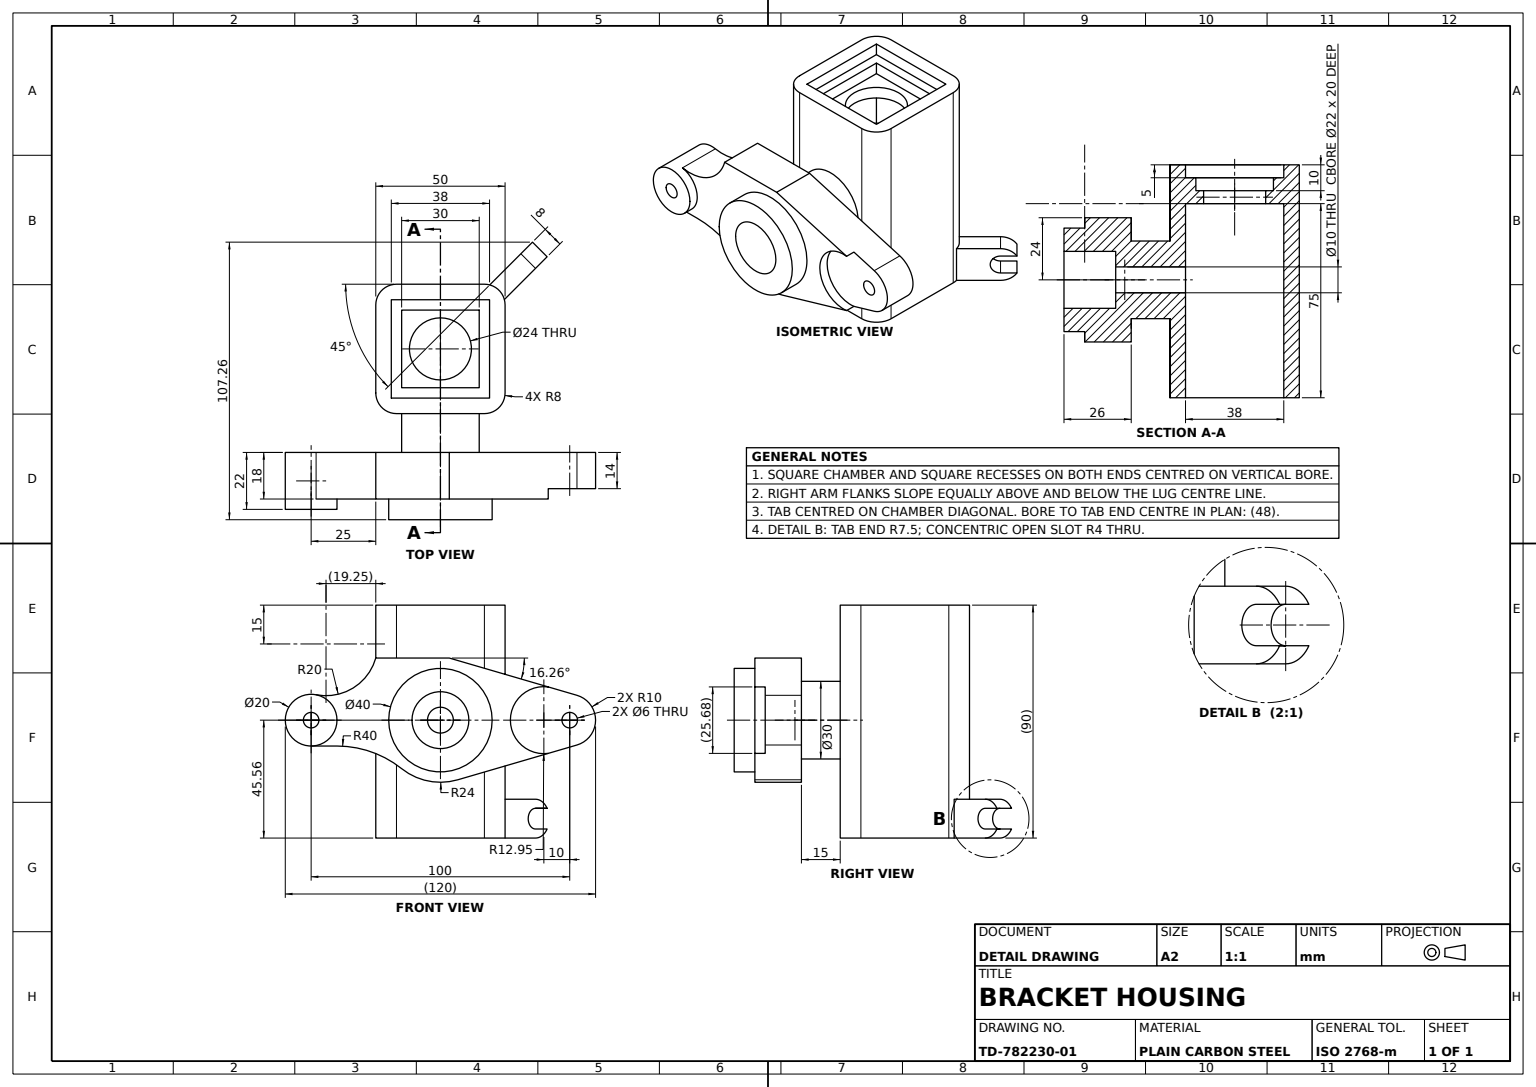
solid
v1 (25,0,17)
v2 (25,0,-17)
e1 v1 v2 LINE
v3 (25,-90,17)
e2 v3 v1 LINE
v4 (25,-90,-17)
e3 v3 v4 LINE
e4 v4 v2 LINE
face PLANE(AX(P(25,-90,17),D(1,0,0),D(0,0,-1))) [-e1 -e2 e3 e4]
v5 (-11,-44.442853,46)
v6 (-11,-44.442853,66)
e5 v5 v6 LINE
v7 (11,-44.442853,66)
e6 v6 v7 CIRCLE(AX(P(0,-44.442853,66),D(0,0,1),D(1,0,0)),11)
v8 (11,-44.442853,46)
e7 v8 v7 LINE
e8 v5 v8 CIRCLE(AX(P(0,-44.442853,46),D(0,0,1),D(1,0,0)),11)
face CYL(AX(P(0,-44.442853,66),D(0,0,1),D(1,0,0)),11) rev [e5 e6 -e7 -e8]
v9 (47,-44.442853,40)
v10 (53,-44.442853,40)
e9 v9 v10 CIRCLE(AX(P(50,-44.442853,40),D(0,0,1),D(1,0,0)),3)
v11 (47,-44.442853,54)
e10 v11 v9 LINE
v12 (53,-44.442853,54)
e11 v11 v12 CIRCLE(AX(P(50,-44.442853,54),D(0,0,1),D(1,0,0)),3)
e12 v12 v10 LINE
face CYL(AX(P(50,-44.442853,54),D(0,0,-1),D(-1,0,0)),3) rev [-e9 -e10 e11 e12]
v13 (-19,-90,-19)
v14 (19,-90,-19)
e13 v13 v14 LINE
v15 (19,-15,-19)
e14 v14 v15 LINE
v16 (-19,-15,-19)
e15 v16 v15 LINE
e16 v13 v16 LINE
face PLANE(AX(P(-19,-90,-19),D(0,0,1),D(1,0,0))) [e13 e14 -e15 -e16]
v17 (-19,0,19)
v18 (19,0,19)
e17 v17 v18 LINE
v19 (19,-5,19)
e18 v19 v18 LINE
v20 (-19,-5,19)
e19 v20 v19 LINE
e20 v20 v17 LINE
face PLANE(AX(P(-19,-5,19),D(0,0,1),D(1,0,0))) rev [e17 -e18 -e19 e20]
v21 (31.112698,-75,-36.769553)
v22 (19.070552,-75,-24.727407)
e21 v21 v22 LINE
v23 (24.727407,-75,-19.070552)
e22 v23 v22 CIRCLE(AX(P(17,-75,-17),D(0,1,0),D(1,0,0)),8)
v24 (36.769553,-75,-31.112698)
e23 v24 v23 LINE
e24 v24 v21 LINE
face PLANE(AX(P(36.769553,-75,-31.112698),D(0,-1,0),D(1,0,0))) rev [e21 -e22 -e23 e24]
v25 (41.255642,-78.5,-35.598788)
e25 v25 v24 CIRCLE(AX(P(36.769553,-82.5,-31.112698),D(0.707106781,0,0.707106781),D(0.707106781,0,-0.707106781)),7.5)
v26 (24.727407,-90,-19.070552)
e26 v23 v26 LINE
v27 (36.769553,-90,-31.112698)
e27 v26 v27 LINE
v28 (41.255642,-86.5,-35.598788)
e28 v27 v28 CIRCLE(AX(P(36.769553,-82.5,-31.112698),D(0.707106781,0,0.707106781),D(0.707106781,0,-0.707106781)),7.5)
v29 (36.769553,-86.5,-31.112698)
e29 v28 v29 LINE
v30 (33.941125,-82.5,-28.284271)
e30 v29 v30 CIRCLE(AX(P(36.769553,-82.5,-31.112698),D(-0.707106781,0,-0.707106781),D(0.707106781,0,-0.707106781)),4)
v31 (36.769553,-78.5,-31.112698)
e31 v30 v31 CIRCLE(AX(P(36.769553,-82.5,-31.112698),D(-0.707106781,0,-0.707106781),D(0.707106781,0,-0.707106781)),4)
e32 v31 v25 LINE
face PLANE(AX(P(36.769553,-82.5,-31.112698),D(0.707106781,0,0.707106781),D(0.707106781,0,-0.707106781))) [e25 e23 e26 e27 e28 e29 e30 e31 e32]
v32 (-53,-44.442853,40)
v33 (-47,-44.442853,40)
e33 v32 v33 CIRCLE(AX(P(-50,-44.442853,40),D(0,0,1),D(1,0,0)),3)
v34 (-53,-44.442853,62)
e34 v34 v32 LINE
v35 (-47,-44.442853,62)
e35 v34 v35 CIRCLE(AX(P(-50,-44.442853,62),D(0,0,1),D(1,0,0)),3)
e36 v35 v33 LINE
face CYL(AX(P(-50,-44.442853,62),D(0,0,-1),D(-1,0,0)),3) rev [-e33 -e34 e35 e36]
v36 (-15,-10,15)
v37 (-15,-10,-15)
e37 v36 v37 LINE
v38 (-15,-5,-15)
e38 v37 v38 LINE
v39 (-15,-5,15)
e39 v38 v39 LINE
e40 v36 v39 LINE
face PLANE(AX(P(-15,-10,15),D(1,0,0),D(0,0,-1))) [e37 e38 e39 -e40]
v40 (19,-5,-19)
e41 v19 v40 LINE
v41 (-19,-5,-19)
e42 v41 v40 LINE
e43 v20 v41 LINE
v42 (15,-5,-15)
e44 v42 v38 LINE
v43 (15,-5,15)
e45 v42 v43 LINE
e46 v43 v39 LINE
face PLANE(AX(P(0,-5,0),D(0,-1,0),D(0,0,-1))) rev [e19 e41 -e42 -e43] [-e44 e45 e46 -e39]
v44 (15,-10,-15)
e47 v44 v42 LINE
v45 (15,-10,15)
e48 v45 v44 LINE
e49 v45 v43 LINE
face PLANE(AX(P(15,-10,15),D(1,0,0),D(0,0,-1))) rev [-e47 -e48 e49 -e45]
v46 (-40,-44.442853,62)
v47 (-40,-44.442853,58)
e50 v46 v47 LINE
v48 (-60,-44.442853,62)
e51 v48 v46 CIRCLE(AX(P(-50,-44.442853,62),D(0,0,1),D(1,0,0)),10)
v49 (-60,-44.442853,40)
e52 v48 v49 LINE
v50 (-50,-54.442853,40)
e53 v49 v50 CIRCLE(AX(P(-50,-44.442853,40),D(0,0,1),D(1,0,0)),10)
v51 (-50,-54.442853,58)
e54 v51 v50 LINE
e55 v51 v47 CIRCLE(AX(P(-50,-44.442853,58),D(0,0,1),D(1,0,0)),10)
face CYL(AX(P(-50,-44.442853,62),D(0,0,-1),D(-1,0,0)),10) [-e50 -e51 e52 e53 -e54 e55]
v52 (31.112698,-90,-36.769553)
e56 v27 v52 LINE
v53 (35.598788,-86.5,-41.255642)
e57 v52 v53 CIRCLE(AX(P(31.112698,-82.5,-36.769553),D(0.707106781,0,0.707106781),D(0.707106781,0,-0.707106781)),7.5)
e58 v28 v53 LINE
face CYL(AX(P(36.769553,-82.5,-31.112698),D(-0.707106781,0,-0.707106781),D(-0.707106781,0,0.707106781)),7.5) [e56 e57 -e58 -e28]
v54 (19.070552,-90,-24.727407)
e59 v22 v54 LINE
v55 (17,-90,-25)
e60 v54 v55 CIRCLE(AX(P(17,-90,-17),D(0,1,0),D(0,0,-1)),8)
v56 (17,0,-25)
e61 v55 v56 LINE
e62 v2 v56 CIRCLE(AX(P(17,0,-17),D(0,1,0),D(0,0,-1)),8)
e63 v4 v26 CIRCLE(AX(P(17,-90,-17),D(0,1,0),D(0,0,-1)),8)
face CYL(AX(P(17,-90,-17),D(0,1,0),D(0,0,1)),8) [-e26 e22 e59 e60 e61 -e62 -e4 e63]
v57 (-17,0,-25)
e64 v56 v57 LINE
v58 (-17,-90,-25)
e65 v55 v58 LINE
e66 v58 v57 LINE
face PLANE(AX(P(-17,-90,-25),D(0,0,-1),D(-1,0,0))) [-e64 -e61 e65 e66]
e67 v10 v9 CIRCLE(AX(P(50,-44.442853,40),D(0,0,1),D(1,0,0)),3)
e68 v33 v32 CIRCLE(AX(P(-50,-44.442853,40),D(0,0,1),D(1,0,0)),3)
v59 (-15,-44.442853,40)
v60 (15,-44.442853,40)
e69 v59 v60 CIRCLE(AX(P(0,-44.442853,40),D(0,0,-1),D(-1,0,0)),15)
e70 v60 v59 CIRCLE(AX(P(0,-44.442853,40),D(0,0,-1),D(-1,0,0)),15)
v61 (52.8,-54.042853,40)
v62 (6.72,-67.482853,40)
e71 v61 v62 LINE
v63 (-14.981238,-63.192853,40)
e72 v63 v62 CIRCLE(AX(P(0,-44.442853,40),D(0,0,1),D(1,0,0)),24)
v64 (-39.949969,-54.442853,40)
e73 v64 v63 CIRCLE(AX(P(-39.949969,-94.442853,40),D(0,0,-1),D(1,0,0)),40)
e74 v50 v64 LINE
v65 (-48.081713,-34.628568,40)
e75 v65 v49 CIRCLE(AX(P(-50,-44.442853,40),D(0,0,1),D(1,0,0)),10)
v66 (-25,-20.442853,40)
e76 v65 v66 CIRCLE(AX(P(-44.245138,-15,40),D(0,0,1),D(1,0,0)),20)
v67 (3.428571,-20.442853,40)
e77 v66 v67 LINE
v68 (52.8,-34.842853,40)
e78 v67 v68 LINE
e79 v61 v68 CIRCLE(AX(P(50,-44.442853,40),D(0,0,1),D(1,0,0)),10)
face PLANE(AX(P(0,0,40),D(0,0,1),D(1,0,0))) rev [e9 e67] [e33 e68] [-e69 -e70] [e71 -e72 -e73 -e74 -e53 -e75 e76 e77 e78 -e79]
v69 (19,0,-19)
e80 v40 v69 LINE
v70 (-19,0,-19)
e81 v70 v69 LINE
e82 v41 v70 LINE
face PLANE(AX(P(-19,-5,-19),D(0,0,1),D(1,0,0))) [e80 -e81 -e82 e42]
e83 v37 v44 LINE
face PLANE(AX(P(-15,-10,-15),D(0,0,1),D(1,0,0))) [e83 e47 e44 -e38]
v71 (-25,-90,17)
v72 (-25,0,17)
e84 v71 v72 LINE
v73 (-17,-90,25)
e85 v71 v73 CIRCLE(AX(P(-17,-90,17),D(0,1,0),D(0,0,-1)),8)
v74 (-17,0,25)
e86 v73 v74 LINE
e87 v72 v74 CIRCLE(AX(P(-17,0,17),D(0,1,0),D(0,0,-1)),8)
face CYL(AX(P(-17,-90,17),D(0,1,0),D(0,0,1)),8) [-e84 e85 e86 -e87]
e88 v35 v34 CIRCLE(AX(P(-50,-44.442853,62),D(0,0,1),D(1,0,0)),3)
face CYL(AX(P(-50,-44.442853,62),D(0,0,-1),D(-1,0,0)),3) rev [-e36 e88 e34 -e68]
e89 v17 v70 LINE
e90 v18 v69 LINE
v75 (17,0,25)
e91 v74 v75 LINE
e92 v75 v1 CIRCLE(AX(P(17,0,17),D(0,1,0),D(0,0,1)),8)
v76 (-25,0,-17)
e93 v57 v76 CIRCLE(AX(P(-17,0,-17),D(0,1,0),D(0,0,-1)),8)
e94 v76 v72 LINE
face PLANE(AX(P(-17,0,17),D(0,-1,0),D(0,0,-1))) rev [-e17 e89 e81 -e90] [e87 e91 e92 e1 e62 e64 e93 e94]
v77 (20,-44.442853,66)
v78 (-20,-44.442853,66)
e95 v77 v78 CIRCLE(AX(P(0,-44.442853,66),D(0,0,-1),D(-1,0,0)),20)
e96 v78 v77 CIRCLE(AX(P(0,-44.442853,66),D(0,0,-1),D(-1,0,0)),20)
e97 v7 v6 CIRCLE(AX(P(0,-44.442853,66),D(0,0,1),D(1,0,0)),11)
face PLANE(AX(P(0,-44.442853,66),D(0,0,-1),D(-1,0,0))) rev [-e95 -e96] [-e97 -e6]
v79 (0,-10,12)
v80 (0,-10,-12)
e98 v79 v80 CIRCLE(AX(P(0,-10,0),D(0,1,0),D(0,0,1)),12)
e99 v80 v79 CIRCLE(AX(P(0,-10,0),D(0,1,0),D(0,0,1)),12)
e100 v36 v45 LINE
face PLANE(AX(P(0,-10,0),D(0,1,0),D(0,0,1))) [-e98 -e99] [-e83 -e37 e100 e48]
v81 (41.6898,-57.283327,58)
v82 (41.6898,-57.283327,54)
e101 v81 v82 LINE
v83 (6.72,-67.482853,58)
e102 v81 v83 LINE
e103 v83 v62 LINE
v84 (52.8,-54.042853,54)
e104 v84 v61 LINE
e105 v84 v82 LINE
face PLANE(AX(P(18.666239,-63.998533,58),D(0.28,-0.96,0),D(0.96,0.28,0))) [-e101 e102 e103 -e71 -e104 e105]
v85 (17,-90,25)
e106 v85 v3 CIRCLE(AX(P(17,-90,17),D(0,1,0),D(0,0,1)),8)
e107 v85 v75 LINE
face CYL(AX(P(17,-90,17),D(0,1,0),D(0,0,1)),8) [e106 e2 -e92 -e107]
v86 (-25,-90,-17)
e108 v58 v86 CIRCLE(AX(P(-17,-90,-17),D(0,1,0),D(0,0,-1)),8)
e109 v86 v76 LINE
face CYL(AX(P(-17,-90,-17),D(0,1,0),D(0,0,1)),8) [-e93 -e66 e108 e109]
v87 (27.048814,-44.442853,54)
e110 v87 v82 CIRCLE(AX(P(40,-44.442853,54),D(0,0,1),D(1,0,0)),12.951186)
v88 (27.048814,-44.442853,58)
e111 v88 v87 LINE
e112 v88 v81 CIRCLE(AX(P(40,-44.442853,58),D(0,0,1),D(1,0,0)),12.951186)
face CYL(AX(P(40,-44.442853,58),D(0,0,-1),D(-1,0,0)),12.951186) rev [e101 -e110 -e111 e112]
v89 (31.112698,-86.5,-36.769553)
e113 v53 v89 LINE
e114 v29 v89 LINE
face PLANE(AX(P(36.769553,-86.5,-31.112698),D(0,-1,0),D(0,0,-1))) rev [-e29 e58 e113 -e114]
v90 (-5,-44.442853,19)
v91 (-5,-44.442853,46)
e115 v90 v91 LINE
v92 (5,-44.442853,46)
e116 v91 v92 CIRCLE(AX(P(0,-44.442853,46),D(0,0,1),D(1,0,0)),5)
v93 (5,-44.442853,19)
e117 v93 v92 LINE
e118 v90 v93 CIRCLE(AX(P(0,-44.442853,19),D(0,0,1),D(1,0,0)),5)
face CYL(AX(P(0,-44.442853,66),D(0,0,1),D(1,0,0)),5) rev [e115 e116 -e117 -e118]
e119 v92 v91 CIRCLE(AX(P(0,-44.442853,46),D(0,0,1),D(1,0,0)),5)
e120 v8 v5 CIRCLE(AX(P(0,-44.442853,46),D(0,0,1),D(1,0,0)),11)
face PLANE(AX(P(5,-44.442853,46),D(0,0,-1),D(-1,0,0))) rev [-e116 -e119] [e8 e120]
v94 (20,-44.442853,58)
v95 (-20,-44.442853,58)
e121 v94 v95 CIRCLE(AX(P(0,-44.442853,58),D(0,0,1),D(1,0,0)),20)
e122 v78 v95 LINE
e123 v77 v94 LINE
face CYL(AX(P(0,-44.442853,66),D(0,0,-1),D(-1,0,0)),20) [e121 -e122 e96 e123]
v96 (41.6898,-31.602378,54)
e124 v96 v87 CIRCLE(AX(P(40,-44.442853,54),D(0,0,1),D(1,0,0)),12.951186)
v97 (41.6898,-31.602378,58)
e125 v97 v96 LINE
e126 v97 v88 CIRCLE(AX(P(40,-44.442853,58),D(0,0,1),D(1,0,0)),12.951186)
face CYL(AX(P(40,-44.442853,58),D(0,0,-1),D(-1,0,0)),12.951186) rev [-e124 -e125 e126 e111]
face CYL(AX(P(0,-44.442853,66),D(0,0,1),D(1,0,0)),11) rev [-e120 e7 e97 -e5]
e127 v12 v11 CIRCLE(AX(P(50,-44.442853,54),D(0,0,1),D(1,0,0)),3)
v98 (52.8,-34.842853,54)
e128 v84 v98 CIRCLE(AX(P(50,-44.442853,54),D(0,0,1),D(1,0,0)),10)
e129 v96 v98 LINE
face PLANE(AX(P(0,0,54),D(0,0,1),D(1,0,0))) [-e127 -e11] [e110 -e105 e128 -e129 e124]
v99 (35.598788,-78.5,-41.255642)
e130 v25 v99 LINE
e131 v99 v21 CIRCLE(AX(P(31.112698,-82.5,-36.769553),D(0.707106781,0,0.707106781),D(0.707106781,0,-0.707106781)),7.5)
face CYL(AX(P(36.769553,-82.5,-31.112698),D(-0.707106781,0,-0.707106781),D(-0.707106781,0,0.707106781)),7.5) [-e25 e130 e131 -e24]
v100 (31.112698,-78.5,-36.769553)
e132 v31 v100 LINE
e133 v100 v99 LINE
face PLANE(AX(P(36.769553,-78.5,-31.112698),D(0,1,0),D(0,0,1))) rev [e132 e133 -e130 -e32]
v101 (15,-44.442853,25)
e134 v101 v60 LINE
v102 (-15,-44.442853,25)
e135 v101 v102 CIRCLE(AX(P(0,-44.442853,25),D(0,0,1),D(1,0,0)),15)
e136 v102 v59 LINE
face CYL(AX(P(0,-44.442853,-17.426407),D(0,0,1),D(1,0,0)),15) [-e134 e135 e136 e69]
e137 v95 v94 CIRCLE(AX(P(0,-44.442853,58),D(0,0,1),D(1,0,0)),20)
face CYL(AX(P(0,-44.442853,66),D(0,0,-1),D(-1,0,0)),20) [e122 e137 -e123 e95]
e138 v86 v71 LINE
face PLANE(AX(P(-25,-90,17),D(-1,0,0),D(0,0,1))) [-e94 -e109 e138 e84]
v103 (0,-15,12)
e139 v103 v79 LINE
v104 (0,-15,-12)
e140 v104 v80 LINE
e141 v103 v104 CIRCLE(AX(P(0,-15,0),D(0,1,0),D(0,0,1)),12)
face CYL(AX(P(0,-15,0),D(0,1,0),D(0,0,1)),12) rev [e139 e98 -e140 -e141]
v105 (3.428571,-20.442853,58)
e142 v105 v97 LINE
v106 (-25,-20.442853,58)
e143 v106 v105 LINE
v107 (-48.081713,-34.628568,58)
e144 v107 v106 CIRCLE(AX(P(-44.245138,-15,58),D(0,0,1),D(1,0,0)),20)
e145 v47 v107 CIRCLE(AX(P(-50,-44.442853,58),D(0,0,1),D(1,0,0)),10)
v108 (-39.949969,-54.442853,58)
e146 v51 v108 LINE
v109 (-14.981238,-63.192853,58)
e147 v108 v109 CIRCLE(AX(P(-39.949969,-94.442853,58),D(0,0,-1),D(1,0,0)),40)
e148 v109 v83 CIRCLE(AX(P(0,-44.442853,58),D(0,0,1),D(1,0,0)),24)
face PLANE(AX(P(0,0,58),D(0,0,1),D(1,0,0))) [-e137 -e121] [-e102 -e112 -e126 -e142 -e143 -e144 -e145 -e55 e146 e147 e148]
e149 v54 v52 LINE
e150 v73 v85 LINE
v110 (-19,-90,19)
e151 v110 v13 LINE
v111 (19,-90,19)
e152 v110 v111 LINE
e153 v111 v14 LINE
face PLANE(AX(P(-17,-90,17),D(0,-1,0),D(0,0,-1))) [-e108 -e65 -e60 e149 -e56 -e27 -e63 -e3 -e106 -e150 -e85 -e138] [-e13 -e151 e152 e153]
e154 v46 v48 CIRCLE(AX(P(-50,-44.442853,62),D(0,0,1),D(1,0,0)),10)
e155 v107 v65 LINE
face CYL(AX(P(-50,-44.442853,62),D(0,0,-1),D(-1,0,0)),10) [-e154 e50 e145 e155 e75 -e52]
face PLANE(AX(P(-19,-5,19),D(1,0,0),D(0,0,-1))) [-e20 e43 e82 -e89]
e156 v109 v63 LINE
e157 v108 v64 LINE
face CYL(AX(P(-39.949969,-94.442853,58),D(0,0,-1),D(-1,0,0)),40) rev [-e156 -e147 e157 e73]
e158 v93 v90 CIRCLE(AX(P(0,-44.442853,19),D(0,0,1),D(1,0,0)),5)
face CYL(AX(P(0,-44.442853,66),D(0,0,1),D(1,0,0)),5) rev [e119 -e115 -e158 e117]
face CYL(AX(P(50,-44.442853,54),D(0,0,-1),D(-1,0,0)),3) rev [e127 e10 -e67 -e12]
v112 (28.284271,-82.5,-33.941125)
e159 v30 v112 LINE
e160 v112 v100 CIRCLE(AX(P(31.112698,-82.5,-36.769553),D(-0.707106781,0,-0.707106781),D(0.707106781,0,-0.707106781)),4)
face CYL(AX(P(36.769553,-82.5,-31.112698),D(-0.707106781,0,-0.707106781),D(-0.707106781,0,0.707106781)),4) rev [e159 e160 -e132 -e31]
e161 v104 v103 CIRCLE(AX(P(0,-15,0),D(0,1,0),D(0,0,1)),12)
face CYL(AX(P(0,-15,0),D(0,1,0),D(0,0,1)),12) rev [-e139 -e161 e140 e99]
e162 v98 v68 LINE
e163 v105 v67 LINE
face PLANE(AX(P(-5.226239,-17.918533,58),D(0.28,0.96,0),D(-0.96,0.28,0))) [e129 e162 -e78 -e163 e142 e125]
v113 (-19,-15,19)
v114 (19,-15,19)
e164 v113 v114 LINE
e165 v111 v114 LINE
e166 v110 v113 LINE
face PLANE(AX(P(-19,-90,19),D(0,0,1),D(1,0,0))) rev [e158 e118] [e164 -e165 -e152 e166]
e167 v89 v112 CIRCLE(AX(P(31.112698,-82.5,-36.769553),D(-0.707106781,0,-0.707106781),D(0.707106781,0,-0.707106781)),4)
face CYL(AX(P(36.769553,-82.5,-31.112698),D(-0.707106781,0,-0.707106781),D(-0.707106781,0,0.707106781)),4) rev [-e30 e114 e167 -e159]
e168 v113 v16 LINE
face PLANE(AX(P(-19,-90,19),D(1,0,0),D(0,0,-1))) [e16 -e168 -e166 e151]
e169 v114 v15 LINE
face PLANE(AX(P(0,-15,0),D(0,-1,0),D(0,0,-1))) [e141 e161] [e168 e15 -e169 -e164]
face CYL(AX(P(50,-44.442853,54),D(0,0,-1),D(-1,0,0)),10) [-e128 e104 e79 -e162]
face PLANE(AX(P(31.112698,-82.5,-36.769553),D(0.707106781,0,0.707106781),D(0.707106781,0,-0.707106781))) rev [-e149 -e59 -e21 -e131 -e133 -e160 -e167 -e113 -e57]
face PLANE(AX(P(-15,-10,15),D(0,0,1),D(1,0,0))) rev [e40 -e46 -e49 -e100]
face PLANE(AX(P(0,0,62),D(0,0,1),D(1,0,0))) [e51 e154] [-e35 -e88]
face PLANE(AX(P(19,-5,19),D(1,0,0),D(0,0,-1))) rev [-e41 e18 e90 -e80]
face PLANE(AX(P(19,-90,19),D(1,0,0),D(0,0,-1))) rev [-e153 e165 e169 -e14]
face CYL(AX(P(0,-44.442853,58),D(0,0,-1),D(-1,0,0)),24) [-e103 -e148 e156 e72]
e170 v102 v101 CIRCLE(AX(P(0,-44.442853,25),D(0,0,1),D(1,0,0)),15)
face CYL(AX(P(0,-44.442853,-17.426407),D(0,0,1),D(1,0,0)),15) [e170 e134 e70 -e136]
face PLANE(AX(P(-17,-90,25),D(0,0,1),D(1,0,0))) [e107 -e91 -e86 e150] [-e170 -e135]
face PLANE(AX(P(0,-54.442853,58),D(0,1,0),D(0,0,1))) rev [-e146 e54 e74 -e157]
e171 v106 v66 LINE
face PLANE(AX(P(0,-20.442853,58),D(0,1,0),D(0,0,1))) [e143 e163 -e77 -e171]
face CYL(AX(P(-44.245138,-15,58),D(0,0,-1),D(-1,0,0)),20) rev [e171 -e76 -e155 e144]
